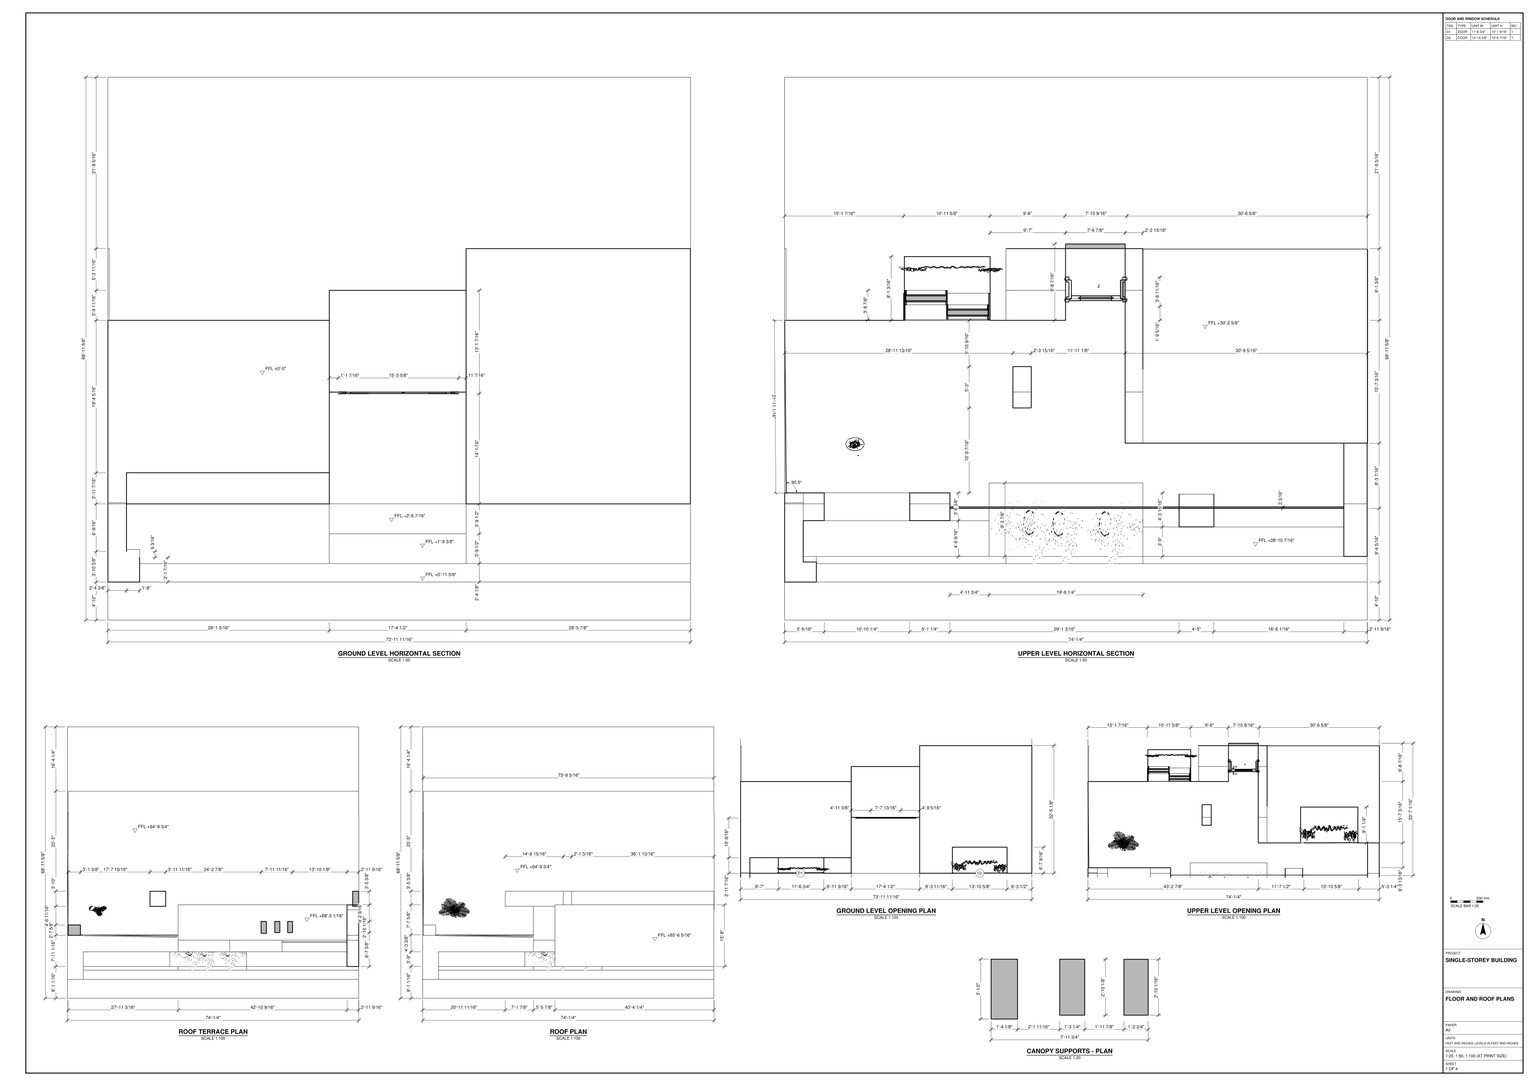
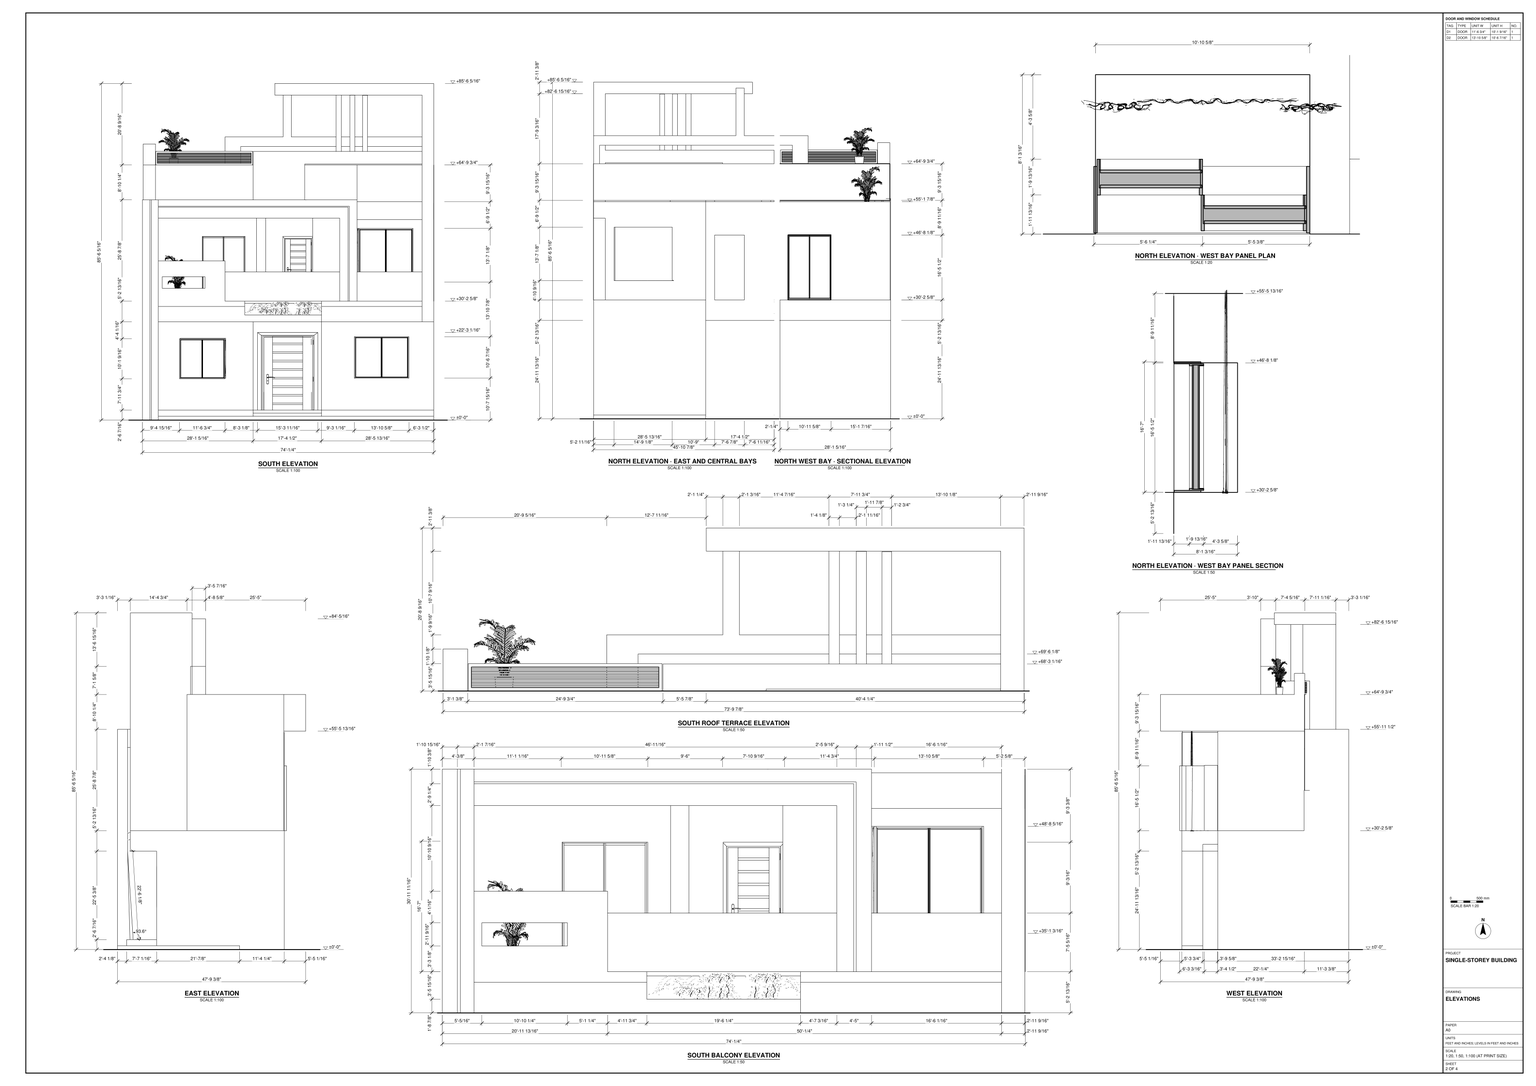
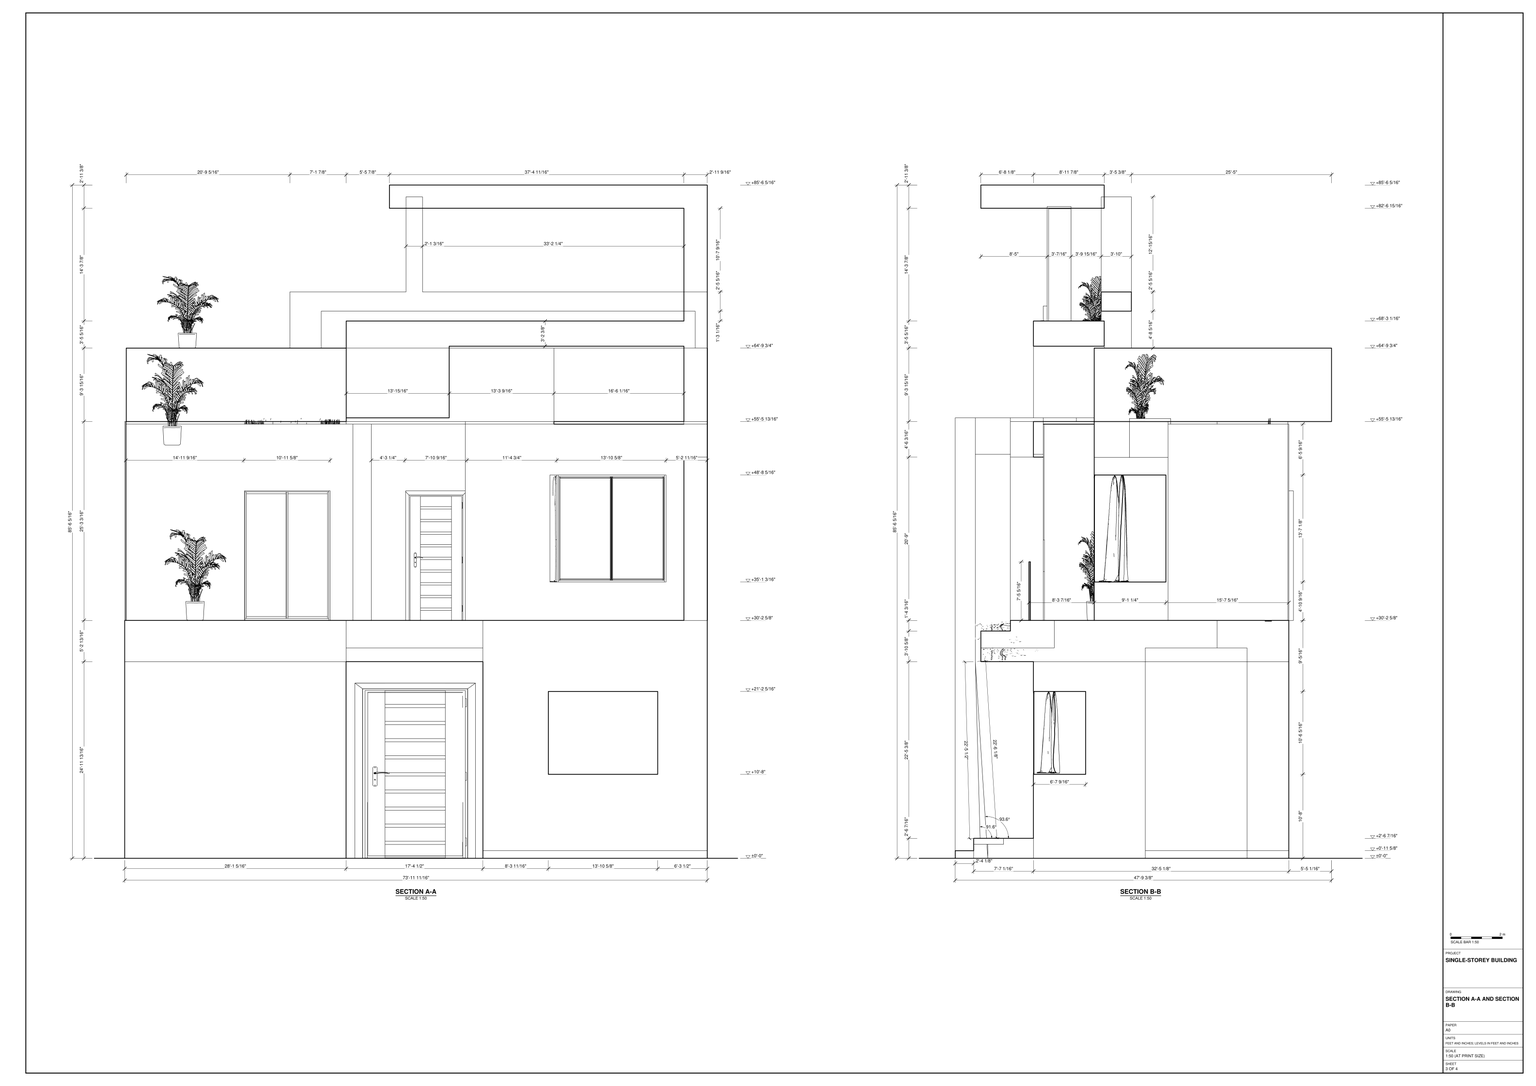
Build the house in SketchUp from task_files/diagram_01.pdf. Work in feet and inches, with the ground floor at ±0'-0". The overall model extents are 305'-8 9/16" along X, 356'-11 1/16" along Y and 85'-6 5/16" along Z. Use the dimensioned horizontal sections to lay out the building footprint and the setbacks between its bays.

Model the walls at the thicknesses drawn, the stepped entrance approach, the floor slabs and the flat roof. On the south elevation, place the framed entrance between the ground-floor windows. Above it, set the upper door and glazed openings behind the balcony. Follow the balcony detail for the projecting rectangular surround, the change in parapet height, the opening through the parapet and the planter above the entrance. Use the roof plan and sections to position the terrace parapet, horizontal screen and raised canopy with its slender supports.

Keep shell elements such as walls, slabs and roof, and each furniture or joinery piece, in separate groups or components; use components for repeated parts. Decor and loose items, including the terrace plants, may be any suitable library components, for example from 3D Warehouse. Save one SketchUp model as output_files/house_with_its_south_balcony_and_roof_terrace.skp.

# SketchUp Ruby script. Lengths in inches.
U = 1.inch
M = Sketchup.active_model
def pt(a) = Geom::Point3d.new(a.map { |v| v * U })
def face(e, loops, mat)
  f = e.add_face(loops[0].map { |a| pt(a) })
  loops[1..].each { |l| e.add_face(l.map { |a| pt(a) }).erase! }
  f.material = f.back_material = mat if mat
  f
end
# faces: each face lists its corners as indices into pts; further lists are holes
def faces(e, pts, list, mat = nil) = list.each { |f| face(e, (f[0].is_a?(Array) ? f : [f]).map { |l| l.map { |i| pts[i] } }, mat) }
# xy, xz, yz: faces in a plane at the given z, y or x. An outline is a flat list of corners, or four numbers for a rectangle; further outlines are holes
def ring(l) = l.size == 4 ? [[l[0], l[1]], [l[2], l[1]], [l[2], l[3]], [l[0], l[3]]] : l.each_slice(2).to_a
def flat(e, list, mat, &to3) = list.each { |f| face(e, (f[0].is_a?(Array) ? f : [f]).map { |l| ring(l).map { |u, v| to3.(u, v) } }, mat) }
def xy(e, z, list, mat = nil) = flat(e, list, mat) { |x, y| [x, y, z] }
def xz(e, y, list, mat = nil) = flat(e, list, mat) { |x, z| [x, y, z] }
def yz(e, x, list, mat = nil) = flat(e, list, mat) { |y, z| [x, y, z] }
def lines(e, pts, list) = list.each { |a, b| e.add_line(pt(pts[a]), pt(pts[b])) }
# prism: a flat outline (further loops are holes) pulled along v
def prism(e, loops, v, mat = nil)
  f = face(e, loops, mat); d = Geom::Vector3d.new(v.map { |x| x * U })
  f.pushpull(f.normal.samedirection?(d) ? d.length : -d.length)
end
def box(e, o, s, mat = nil) = prism(e, [[o, [o[0] + s[0], o[1], o[2]], [o[0] + s[0], o[1] + s[1], o[2]], [o[0], o[1] + s[1], o[2]]]], [0, 0, s[2]], mat)
def at(x, y, z, deg = 0) = Geom::Transformation.translation(pt([x, y, z])) * Geom::Transformation.rotation(ORIGIN, Z_AXIS, deg.degrees)
def axes(o, x, y, z) = Geom::Transformation.new([*x, 0, *y, 0, *z, 0, *pt(o).to_a, 1])
def part(name) = M.definitions.add(name)
# library, detail: a bought-in or finely detailed component or shape, given as its bounding box
def library(name, o, s) = part(name).tap { |d| box(d.entities, o, s) }
def detail(e, o, s) = box(e.add_group.entities, o, s)
def put(e, d, t, mat = nil) = e.add_instance(d, t).tap { |i| i.material = mat if mat }
def group(e, t, mat = nil) = e.add_group.tap { |g| g.transformation = t; g.material = mat if mat }.entities
root = M.entities
M.materials.add("Glass_Tinted_Gray").color = [0, 0, 0]
M.materials["Glass_Tinted_Gray"].alpha = 0.125
M.materials.add("Material~14").color = [247, 247, 247]
M.materials.add("Material~2").color = [49, 49, 49]
M.materials.add("Material~6").color = [130, 95, 63]
M.materials.add("Niraj_Hair_Dark").color = [109, 109, 109]
M.materials.add("[0135_DarkGray]").color = [81, 81, 81]
M.materials.add("[Asphalt_New]").color = [58, 58, 58]
M.materials.add("[Color C01]").color = [255, 229, 204]
M.materials.add("[Color M00]").color = [255, 255, 255]
M.materials.add("[Mirror 02]").color = [229, 229, 229]
M.materials.add("[Mirror 02]1").color = [229, 229, 229]
M.materials.add("[Terrazzo Light Blue]").color = [196, 214, 227]
c1 = library("curtian",[-4.5,-7.8,0.05],[158.46,10.43,112.21])
c2 = part("PENTEK_RP Fineline 50S_Sliding_DoorCase_E1")
box(c2.entities,[0,0,0],[1.51,3.66,99.27],"[0135_DarkGray]")
c3 = part("PENTEK_RP Fineline 50S_SlidingDooe_Case_E2")
box(c3.entities,[0,0,0],[96.25,3.66,1.51],"[0135_DarkGray]")
c4 = part("pentek_RP Fineline 50S_SlidingDoor_Case")
put(c4.entities,c2,at(97.76,0,0))
put(c4.entities,c3,at(1.51,0,0))
put(c4.entities,c2,at(0,0,0))
put(c4.entities,c3,at(1.51,0,97.76))
c5 = part("PENTEK_RP Fineline 50S_SlidingDoor_GlazingBead_2")
box(c5.entities,[0,0,0],[0.56,0.59,94.39],"[0135_DarkGray]")
c6 = part("PENTEK_RP Fineline 50S_SlidingDoor_Glass")
box(c6.entities,[0,0,0],[46.58,0.16,94.39],"Glass_Tinted_Gray")
c7 = part("PENTEK_RP Fineline 50S_SlidingDoor_GlazingBead")
box(c7.entities,[0,0,0],[45.47,0.59,0.56],"[0135_DarkGray]")
c8 = part("PENTEK_RP Fineline 50S_SlidingDoor_Leaf_E1")
xy(c8.entities,0,[[0,0,0.93,1.97],[0.93,1.57,1.49,1.97]],"[0135_DarkGray]")
xy(c8.entities,96.25,[[0,0,0.93,0,0.93,1.57,1.49,1.57,1.49,1.97,0,1.97]],"[0135_DarkGray]")
xz(c8.entities,0,[[0,0,0.93,96.25]],"[0135_DarkGray]")
xz(c8.entities,1.57,[[0.93,0,1.49,95.32],[0.93,95.32,1.49,96.25]],"[0135_DarkGray]")
xz(c8.entities,1.97,[[0,0,1.49,96.25]],"[0135_DarkGray]")
yz(c8.entities,0,[[0,0,1.97,96.25]],"[0135_DarkGray]")
yz(c8.entities,0.93,[[0,0,1.57,0.93],[0,0.93,1.57,95.32],[0,95.32,1.57,96.25]],"[0135_DarkGray]")
yz(c8.entities,1.49,[[1.57,0,1.97,95.32],[1.57,95.32,1.97,96.25]],"[0135_DarkGray]")
c9 = part("PENTEK_RP Fineline 50S_SlidingDoor_Leaf_E2")
xy(c9.entities,0,[[0,0,0,1.57,0.56,1.57,0.56,1.97,46.02,1.97,46.02,1.57,46.58,1.57,46.58,0]],"[0135_DarkGray]")
xy(c9.entities,0.93,[[0,0,46.58,1.57]],"[0135_DarkGray]")
xy(c9.entities,1.49,[[0.56,1.57,46.02,1.97]],"[0135_DarkGray]")
xz(c9.entities,0,[[0,0,46.58,0.93]],"[0135_DarkGray]")
xz(c9.entities,1.57,[[0,0,0.56,0.93],[46.02,0,46.58,0.93],[0.56,0.93,46.02,1.49]],"[0135_DarkGray]")
xz(c9.entities,1.97,[[0.56,0,46.02,1.49]],"[0135_DarkGray]")
yz(c9.entities,0,[[0,0,1.57,0.93]],"[0135_DarkGray]")
yz(c9.entities,0.56,[[1.57,0,1.97,0.93],[1.57,0.93,1.97,1.49]],"[0135_DarkGray]")
yz(c9.entities,46.02,[[1.57,0,1.97,0.93],[1.57,0.93,1.97,1.49]],"[0135_DarkGray]")
yz(c9.entities,46.58,[[0,0,1.57,0.93]],"[0135_DarkGray]")
c10 = part("PENTEK_RP Fineline S_SlidingDoor_Leaf1")
put(c10.entities,c5,at(0.93,0,0.93))
put(c10.entities,c5,at(46.96,0,0.93))
put(c10.entities,c6,at(1.49,1.42,0.93))
put(c10.entities,c7,at(1.49,0,0.93))
put(c10.entities,c6,at(1.49,0.59,0.93),"[Terrazzo Light Blue]")
put(c10.entities,c8,at(0,0,0))
put(c10.entities,c8,axes([48.44,0,0],[-1,0,0],[0,1,0],[0,0,1]))
put(c10.entities,c9,axes([0.93,0,96.25],[1,0,0],[0,1,0],[0,0,-1]))
put(c10.entities,c9,at(0.93,0,0))
put(c10.entities,c7,at(1.49,0,94.77))
c11 = part("PENTEK_RP Fineline 50S_SlidingDoor_Leaf2")
put(c11.entities,c6,at(1.49,1.42,0.93))
put(c11.entities,c7,at(1.49,0,94.77))
put(c11.entities,c5,at(46.96,0,0.93))
put(c11.entities,c6,at(1.49,0.59,0.93),"[Mirror 02]")
put(c11.entities,c5,at(0.93,0,0.93))
put(c11.entities,c8,at(0,0,0))
put(c11.entities,c8,axes([48.44,0,0],[-1,0,0],[0,1,0],[0,0,1]))
put(c11.entities,c7,at(1.49,0,0.93))
put(c11.entities,c9,axes([0.93,0,96.25],[1,0,0],[0,1,0],[0,0,-1]))
put(c11.entities,c9,at(0.93,0,0))
c12 = part("PENTEK - Slimmest Steel Sliding Door / Window\#1")
put(c12.entities,c4,at(0,-1.88,-0.09))
put(c12.entities,c10,at(1.51,-2.27,1.42))
put(c12.entities,c11,at(49.32,-0.3,1.42))
c13 = library("Group6\#1",[-22.44,-5.97,0],[42.52,9.29,84.25])
c14 = library("TS_VASO+GANCHOS-PARA-PENDURAR\#1",[-17.61,-15.74,-70.29],[36.55,50.24,77.96])
c15 = library("3D Plant 003",[-20.34,-12.34,-8.74],[41.02,24.08,18.2])
c16 = library("SKT_Nearly Natural 5' Kentia Palm Silk Tree",[-23.18,-17.61,0],[47.48,43.95,59.125])
c17 = part("Glass Door - Open Shower")
box(c17.entities,[0,0,0.95],[40,1.5,72])
c18 = part("Glass")
put(c18.entities,c17,axes([-0.67,0,24.24],[0,0,-0.606],[0,1,0],[0.69991,0,0]),"[Mirror 02]1")
c19 = library("Sphere Light",[-16.25,-16.25,-16.25],[32.5,32.5,32.5])
c20 = library("Sphere Light\#1",[-11.51,-11.51,-11.51],[23.02,23.02,23.02])
c21 = library("Sphere Light\#2",[-4.58,-4.58,-4.58],[9.16,9.16,9.16])
c22 = library("Sphere Light\#3",[-9.0625,-9.0625,-9.0625],[18.125,18.125,18.125])
c23 = library("Sphere Light\#4",[-6.43,-6.43,-6.43],[12.86,12.86,12.86])
c24 = library("Sphere Light\#5",[-6.71,-6.71,-6.71],[13.42,13.42,13.42])
c25 = library("Sphere Light\#6",[-9.57,-9.57,-9.57],[19.14,19.14,19.14])
c26 = library("Sphere Light\#7",[-21.77,-21.77,-21.77],[43.54,43.54,43.54])
c27 = library("Sphere Light\#8",[-25.16,-25.16,-25.16],[50.32,50.32,50.32])
c28 = library("Dome Light",[-12,-12,0],[24,24,12])
c29 = library("Dome Light\#1",[-12,-12,0],[24,24,12])
c30 = library("Dome Light\#2",[-12,-12,0],[24,24,12])
xy(root,0,[[0,0,3668.5625,4283.0625],[1460.375,2111.35,2348.05,2169.35],[1460.375,2169.35,2348.05,2169.35,2348.05,2677.67,2006.2,2677.67,2006.2,2288.52,1460.375,2288.52],[1460.375,2288.52,1488.72,2290.35],[1488.72,2288.52,1797.7,2288.52,1797.7,2568.29,1460.375,2568.29,1460.375,2290.35,1488.72,2290.35],
  [1797.7,2288.52,2006.2,2458.93],[1460.375,2568.29,1462.375,2677.67],[1462.375,2568.29,1797.7,2568.29,1797.7,2613.99,2006.2,2613.99,2006.2,2677.67,2348.05,2677.67,2348.05,2938.98,1460.375,2938.98,1460.375,2677.67,1462.375,2677.67]])
xy(root,11.625,[[1508.72,2169.35,2348.05,2197.47]])
xy(root,21.375,[[1797.7,2197.47,2006.2,2243]])
xy(root,30.4375,[[1508.72,2197.47,1797.7,2197.47,1797.7,2335.95,1488.72,2335.95,1488.72,2218.98,1508.72,2218.98],[2006.2,2197.47,2348.05,2288.52],[1797.7,2243,2006.2,2288.52]])
xy(root,128.03,[[1575.39,2288.52,1714.14,2335.95],[2105.92,2288.52,2272.54,2368.1]])
xy(root,249.53,[[1575.39,2288.52,1714.14,2335.95]])
xy(root,254.34,[[2105.92,2288.52,2272.54,2368.1]])
xy(root,299.8125,[[1488.72,2208.39,1797.7,2288.52],[1797.7,2208.39,2006.2,2677.67],[2006.2,2208.39,2068.96,2288.52],[2068.96,2208.39,2107.78,2288.52],[2107.78,2208.39,2348.05,2288.52],
  [1488.72,2288.52,1797.7,2335.95]])
xy(root,320.6875,[[1771.95,2208.39,2006.2,2320.29],[1797.7,2458.93,2006.2,2613.99]])
xy(root,346.43,[[1488.72,2208.39,1771.95,2262.95],[2006.2,2208.39,2312.46,2253.39]])
xy(root,362.625,[[[2006.2,2253.39,2061.4,2253.39,2061.4,2303.45,2114.41,2303.45,2114.41,2253.39,2312.46,2253.39,2312.46,2381.11,1979.26,2381.11,1979.26,2684.73,1888.39,2684.73,1888.39,2568.29,1460.375,2568.29,1462.74,2305.32,1712.19,2305.32,1712.19,2262.95,1771.95,2262.95,1771.95,2320.29,2006.2,2320.29],[1808.19,2434.75,1836.13,2497.75]],[2061.4,2253.39,2114.41,2303.45],[1460.375,2305.32,1462.74,2305.32,1460.375,2568.29],[2006.2,2381.11,2348.05,2676.24],[2348.05,2381.11,2348.61,2676.24],
  [1642.8,2568.29,1773.42,2665.48],[2006.2,2676.24,2348.05,2677.67]])
xy(root,401.75,[[1520.68,2262.95,1650.9375,2305.32]])
xy(root,421.2,[[2108.27,2381.11,2282.83,2490.36]])
xy(root,437.25,[[1520.68,2262.95,1650.9375,2305.32]])
xy(root,485.3125,[[1488.72,2262.95,1712.19,2262.95,1712.19,2305.32,1460.375,2305.32,1460.375,2290.35,1488.72,2290.35],[1460.375,2288.52,1488.72,2290.35]])
xy(root,560.12,[[1642.8,2568.29,1773.42,2665.48],[1888.39,2568.29,1979.26,2684.73]])
xy(root,584.33,[[2108.27,2381.11,2282.83,2490.36]])
xy(root,611.61,[[2114.41,2288.52,2312.46,2303.45]])
xy(root,661.875,[[2114.41,2303.45,2312.46,2381.11],[1979.26,2493.62,2006.2,2493.62,2006.2,2677.67,1797.7,2677.67,1797.7,2568.29,1979.26,2568.29]])
xy(root,665.8125,[[2114.41,2288.52,2312.46,2381.11],[1462.75,2304.74,1462.75,2742.74,2348.05,2742.74,2348.05,2381.11,1797.9,2381.11,1797.9,2304.74]])
xy(root,670.375,[[1808.19,2434.75,1836.13,2497.75]])
xy(root,671.5,[[1460.375,2169.35,1460.375,2303.45,1797.9,2303.45,1797.9,2253.39,1508.72,2253.39,1508.72,2169.35],[1797.9,2253.39,1954.84,2288.52],[1954.84,2253.39,2114.41,2303.45],[1797.9,2288.52,1954.84,2303.45],[1797.9,2303.45,1954.84,2381.11]])
xy(root,777.75,[[1796.3,2299.59,1501.21,2304.74,1509.71,2304.74,1796.3,2299.73],[1462.75,2303.45,1500.15,2303.45,1462.75,2304.74],[1500.15,2303.45,1462.75,2304.74,1500.15,2304.74],[[1500.15,2304.74,1501.21,2304.74,1501.22,2304.89,1509.71,2304.74,1797.9,2304.74,1797.9,2396.36,1954.84,2396.36,1954.84,2381.11,2312.46,2381.11,2312.46,2396.36,2348.05,2396.36,2348.05,2384.86,2348.61,2384.86,2348.61,2676.24,2348.05,2676.24,2348.05,2742.74,1462.75,2742.74,1462.75,2335.05,1500.15,2335.05],[1712.05,2391.77,1759.8,2437.77]],[1501.21,2304.74,1501.22,2304.89,1509.71,2304.74],
  [1797.9,2381.11,1954.84,2396.36],[2312.46,2381.11,2348.05,2396.36],[2348.05,2381.11,2348.61,2384.86]])
xy(root,777.77,[[2329.69,2391.77,2348.05,2437.77]])
xy(root,780.6875,[[1954.84,2288.52,2312.46,2396.36]])
xy(root,782.77,[[1791.87,2299.66,1791.875,2299.96,1505.64,2304.96,1505.64,2304.66]])
xy(root,782.77,[[1791.83,2297.14,1791.87,2299.66,1505.64,2304.66,1505.6,2302.14]],"Material~2")
xy(root,783.44,[[1791.23,2297.15,1506.19,2302.13,1506.23,2304.8,1791.28,2299.82]],"Material~2")
xy(root,785.24,[[1791.25,2298,1791.28,2299.82,1506.23,2304.8,1506.2,2302.98]],"Material~2")
xy(root,787.03,[[1791.25,2298,1506.2,2302.98,1506.23,2304.8,1791.28,2299.82]],"Material~2")
xy(root,788.82,[[1791.25,2298,1791.28,2299.82,1506.23,2304.8,1506.2,2302.98]],"Material~2")
xy(root,790.62,[[1791.25,2298,1506.2,2302.98,1506.23,2304.8,1791.28,2299.82]],"Material~2")
xy(root,792.41,[[1791.25,2298,1791.28,2299.82,1506.23,2304.8,1506.2,2302.98]],"Material~2")
xy(root,794.2,[[1791.25,2298,1506.2,2302.98,1506.23,2304.8,1791.28,2299.82]],"Material~2")
xy(root,796,[[1791.25,2298,1791.28,2299.82,1506.23,2304.8,1506.2,2302.98]],"Material~2")
xy(root,797.79,[[1791.25,2298,1506.2,2302.98,1506.23,2304.8,1791.28,2299.82]],"Material~2")
xy(root,799.58,[[1791.25,2298,1791.28,2299.82,1506.23,2304.8,1506.2,2302.98]],"Material~2")
xy(root,801.375,[[1791.25,2298,1506.2,2302.98,1506.23,2304.8,1791.28,2299.82]],"Material~2")
xy(root,803.17,[[1791.25,2298,1791.28,2299.82,1506.23,2304.8,1506.2,2302.98]],"Material~2")
xy(root,804.96,[[1791.25,2298,1506.2,2302.98,1506.23,2304.8,1791.28,2299.82]],"Material~2")
xy(root,806.76,[[1791.25,2298,1791.28,2299.82,1506.23,2304.8,1506.2,2302.98]],"Material~2")
xy(root,808.55,[[1791.25,2298,1506.2,2302.98,1506.23,2304.8,1791.28,2299.82]],"Material~2")
xy(root,810.34,[[1791.25,2298,1791.28,2299.82,1506.23,2304.8,1506.2,2302.98]],"Material~2")
xy(root,812.13,[[1791.25,2298,1506.2,2302.98,1506.23,2304.8,1791.28,2299.82]],"Material~2")
xy(root,813.93,[[1791.23,2297.15,1791.28,2299.82,1506.23,2304.8,1506.19,2302.13]],"Material~2")
xy(root,814.6,[[1791.87,2299.66,1505.64,2304.66,1505.64,2304.96,1791.875,2299.96]])
xy(root,814.6,[[1791.83,2297.14,1505.6,2302.14,1505.64,2304.66,1791.87,2299.66]],"Material~2")
xy(root,819.05,[[[1797.9,2288.52,2312.46,2396.36],[2050.64,2309.39,2066.76,2345.89],[2092.45,2311.77,2107.7,2345.89],[2131.62,2311.77,2146.37,2345.83]]])
xy(root,819.62,[[1796.3,2299.59,1796.3,2299.73,1501.22,2304.89,1501.21,2304.74]])
xy(root,834.09,[[1759.8,2391.77,2329.69,2437.77]])
xy(root,841.875,[[1462.75,2303.45,1500.15,2335.05]])
xy(root,863.375,[[1712.05,2391.77,1889.02,2437.77],[1914.2,2391.77,2348.05,2437.77]])
xy(root,990.23,[[2131.62,2311.77,2146.37,2345.83]])
xy(root,990.61,[[2092.45,2311.77,2107.7,2345.89]])
xy(root,990.94,[[1863.78,2208.39,2312.46,2396.36]])
xy(root,993.73,[[2050.64,2309.39,2066.76,2345.89]])
xy(root,1008.3125,[[1889.02,2391.77,1914.2,2437.77]])
xy(root,1026.3125,[[1863.78,2208.39,2348.05,2396.36]])
xz(root,2169.35,[[1483.3,0,1487.83,671.5]])
xz(root,2169.35,[[1460.375,0,1483.3,671.5],[1487.83,0,1508.72,671.5]],"Material~6")
xz(root,2169.35,[[1508.72,0,2348.05,11.625]],"[Color M00]")
xz(root,2197.47,[[1797.7,0,2006.2,11.625],[1508.72,11.625,1797.7,30.4375],[1797.7,11.625,2006.2,21.375],[2006.2,11.625,2348.05,30.4375]])
xz(root,2199.93,[[1488.72,299.8125,1508.72,615.9]])
xz(root,2208.39,[[2312.46,299.8125,2348.05,299.8125,2348.05,1026.3125,1863.78,1026.3125,1863.78,990.94,2312.46,990.94]])
xz(root,2208.39,[[1488.72,299.8125,2006.2,299.8125,2006.2,320.6875,1771.95,320.6875,1771.95,346.43,1488.72,346.43],[2006.2,299.8125,2312.46,346.43]],"Niraj_Hair_Dark")
xz(root,2218.98,[[1488.72,0,1508.72,30.4375]])
xz(root,2243,[[1797.7,21.375,2006.2,30.4375]])
xz(root,2253.39,[[2006.2,346.43,2312.46,362.625],[2087.16,362.625,2090.9375,362.625,2090.9375,651.9375,1508.72,651.9375,1508.72,649.15,2087.16,649.15]])
xz(root,2253.39,[[2061.4,362.625,2087.16,362.625,2087.16,649.15,1508.72,649.15,1508.72,615.9,2061.4,615.9],[2090.9375,362.625,2114.41,362.625,2114.41,671.5,1508.72,671.5,1508.72,651.9375,2090.9375,651.9375]],"Material~6")
xz(root,2262.95,[[[1488.72,346.43,1771.95,346.43,1771.95,362.625,1712.19,362.625,1712.19,485.3125,1488.72,485.3125],[1520.68,401.75,1650.9375,437.25]]])
xz(root,2288.52,[[1797.7,0,1814.75,11.625],[1814.75,0,2006.2,11.625],[[1488.72,11.625,1797.7,299.8125],[1575.39,128.03,1714.14,249.53]],[1797.7,11.625,2006.2,30.4375],[2114.41,611.61,2312.46,665.8125],
  [1797.9,671.5,1954.84,671.5,1954.84,780.6875,2312.46,780.6875,2312.46,819.05,1797.9,819.05]])
xz(root,2288.52,[[[2006.2,30.4375,2348.05,299.8125],[2105.92,128.03,2272.54,254.34]]],"[Color C01]")
xz(root,2303.45,[[1460.375,615.9,1462.375,671.5],[2114.41,665.8125,2114.41,671.5,1954.84,671.5],[1462.75,777.75,1500.15,841.875]])
xz(root,2304.74,[[1462.75,665.8125,1797.9,777.75]],"Niraj_Hair_Dark")
xz(root,2305.32,[[[1460.375,362.625,1712.19,485.3125],[1520.68,401.75,1650.9375,437.25]]])
xz(root,2309.39,[[2050.64,819.05,2066.76,993.73]])
xz(root,2311.77,[[2092.45,819.05,2107.7,990.61],[2131.62,819.05,2146.37,990.23]])
xz(root,2320.29,[[1771.95,320.6875,2006.2,356.29],[1771.95,356.29,2006.2,362.625]])
xz(root,2335.05,[[1462.75,777.75,1500.15,841.875]])
xz(root,2335.95,[[[1488.72,30.4375,1797.7,299.8125],[1575.39,128.03,1714.14,249.53]],[1575.39,128.03,1714.14,249.53]])
xz(root,2345.83,[[2131.62,819.05,2146.37,990.23]])
xz(root,2345.89,[[2050.64,819.05,2066.76,993.73],[2092.45,819.05,2107.7,990.61]])
xz(root,2368.1,[[2105.92,128.03,2272.54,254.34]])
xz(root,2381.11,[[[1979.26,362.625,2312.46,362.625,2312.46,611.61,2347.97,611.61,2347.97,661.875,1979.26,661.875],[2108.27,421.2,2282.83,584.33]],[2312.46,362.625,2348.05,611.61],[2348.05,362.625,2348.61,611.61],[2347.97,611.61,2348.05,661.875],[2348.05,611.61,2348.61,661.875],
  [1797.9,661.875,1979.26,665.8125],[1979.26,661.875,2114.41,665.8125],[2114.41,661.875,2312.46,665.8125],[2312.46,661.875,2348.05,777.75],[2348.05,661.875,2348.61,665.8125],
  [2348.05,665.8125,2348.61,777.75],[1797.9,671.5,1954.84,777.75]])
xz(root,2381.11,[[2114.41,665.8125,2312.46,777.75]],"Material~6")
xz(root,2381.11,[[1797.9,665.8125,2114.41,665.8125,2114.41,777.75,1954.84,777.75,1954.84,671.5,1797.9,671.5]],"Niraj_Hair_Dark")
xz(root,2391.77,[[1712.05,777.75,1759.8,777.75,1759.8,834.09,2329.69,834.09,2329.69,777.77,2348.05,777.77,2348.05,863.375,1914.2,863.375,1914.2,1008.3125,1889.02,1008.3125,1889.02,863.375,1712.05,863.375]],"Niraj_Hair_Dark")
xz(root,2396.36,[[1797.9,777.75,1797.9,819.05,2312.46,819.05,2312.46,990.94,1863.78,990.94,1863.78,1026.3125,2348.05,1026.3125,2348.05,777.75,2312.46,777.75,2312.46,780.6875,1954.84,780.6875,1954.84,777.75]])
xz(root,2434.75,[[1808.19,362.625,1836.13,670.375]])
xz(root,2437.77,[[1712.05,777.75,1712.05,863.375,1889.02,863.375,1889.02,1008.3125,1914.2,1008.3125,1914.2,863.375,2348.05,863.375,2348.05,777.77,2329.69,777.77,2329.69,834.09,1759.8,834.09,1759.8,777.75]])
xz(root,2458.93,[[1797.7,0,2006.2,320.6875]])
xz(root,2490.36,[[2108.27,421.2,2282.83,584.33]])
xz(root,2493.62,[[1979.26,611.0625,2006.2,661.875]])
xz(root,2497.75,[[1808.19,362.625,1836.13,670.375]])
xz(root,2568.29,[[1460.375,0,1797.7,299.8125],[1460.375,299.8125,1797.7,362.625]])
xz(root,2568.29,[[1462.375,362.625,1642.8,362.625,1642.8,560.12,1773.42,560.12,1773.42,362.625,1888.39,362.625,1888.39,560.12,1979.26,560.12,1979.26,661.875,1462.375,661.875]],"[Color C01]")
xz(root,2613.99,[[1797.7,0,2006.2,320.6875]])
xz(root,2665.48,[[1642.8,362.625,1773.42,560.12]])
xz(root,2676.24,[[2348.05,362.625,2348.61,665.8125],[2348.05,665.8125,2348.61,777.75]])
xz(root,2677.67,[[2006.2,0,2348.05,11.625],[2006.2,11.625,2348.05,362.625],[1797.7,299.8125,2006.2,661.875]])
xz(root,2684.73,[[1888.39,362.625,1979.26,560.12]])
xz(root,2742.74,[[1462.75,665.8125,2348.05,777.75]])
yz(root,1460.375,[[2169.35,0,2169.35,671.5,2303.45,671.5,2303.45,485.3125,2305.32,485.3125,2305.32,362.625,2568.29,362.625,2568.29,0]],"Material~14")
yz(root,1462.75,[[2304.74,665.8125,2304.74,777.75,2303.45,777.75,2303.45,841.875,2335.05,841.875,2335.05,777.75,2742.74,777.75,2742.74,665.8125]])
yz(root,1488.72,[[2288.52,0,2290.35,11.625],[2288.52,11.625,2290.35,30.4375],[2288.52,30.4375,2335.95,299.8125]])
yz(root,1488.72,[[2218.98,0,2218.98,30.4375,2288.52,30.4375,2288.52,299.8125,2208.39,299.8125,2208.39,346.43,2262.95,346.43,2262.95,485.3125,2288.52,485.3125,2288.52,615.9,2199.93,615.9,2199.93,299.8125]],"Niraj_Hair_Dark")
yz(root,1500.15,[[2303.45,777.75,2335.05,841.875]])
yz(root,1505.64,[[2304.66,782.77,2304.96,814.6]])
yz(root,1506.2,[[2302.83,785.24,2302.83,785.57,2302.875,785.34,2302.98,785.24],[2302.83,786.7,2302.83,787.03,2302.98,787.03,2302.875,786.93],[2302.83,788.82,2302.83,789.16,2302.875,788.92,2302.98,788.82],[2302.83,790.28,2302.83,790.62,2302.98,790.62,2302.875,790.52],[2302.83,792.41,2302.83,792.75,2302.875,792.51,2302.98,792.41],
  [2302.83,793.87,2302.83,794.2,2302.98,794.2,2302.875,794.11],[2302.83,796,2302.83,796.33,2302.875,796.09,2302.98,796],[2302.83,797.45,2302.83,797.79,2302.98,797.79,2302.875,797.69],[2302.83,799.58,2302.83,799.92,2302.875,799.68,2302.98,799.58],[2302.83,801.04,2302.83,801.375,2302.98,801.375,2302.875,801.28],
  [2302.83,803.17,2302.83,803.5,2302.875,803.27,2302.98,803.17],[2302.83,804.625,2302.83,804.96,2302.98,804.96,2302.875,804.86],[2302.83,806.76,2302.83,807.09,2302.875,806.85,2302.98,806.76],[2302.83,808.21,2302.83,808.55,2302.98,808.55,2302.875,808.45],[2302.83,810.34,2302.83,810.68,2302.875,810.4375,2302.98,810.34],
  [2302.83,811.8,2302.83,812.13,2302.98,812.13,2302.875,812.04]])
yz(root,1508.72,[[2197.47,0,2218.98,0,2217.04,30.4375,2197.47,30.4375],[2218.98,0,2217.04,30.4375,2218.98,30.4375]])
yz(root,1508.72,[[2169.35,11.625,2197.47,11.625,2197.47,30.4375,2207.26,30.4375,2199.93,299.8125,2199.93,671.5,2169.35,671.5],[2199.93,615.9,2253.39,671.5]],"Material~6")
yz(root,1520.68,[[2262.95,401.75,2305.32,437.25]])
yz(root,1575.39,[[2288.52,128.03,2335.95,249.53]])
yz(root,1642.8,[[2568.29,362.625,2665.48,560.12]])
yz(root,1650.9375,[[2262.95,401.75,2305.32,437.25]])
yz(root,1712.05,[[2391.77,777.75,2437.77,863.375]])
yz(root,1712.19,[[2262.95,362.625,2305.32,437.25],[2262.95,437.25,2305.32,485.3125]])
yz(root,1714.14,[[2288.52,128.03,2335.95,249.53]])
yz(root,1759.8,[[2391.77,777.75,2437.77,834.09]])
yz(root,1771.95,[[2208.39,320.6875,2320.29,320.6875,2320.29,356.29,2262.95,356.29,2262.95,346.43,2208.39,346.43],[2262.95,356.29,2320.29,362.625]])
yz(root,1773.42,[[2568.29,362.625,2665.48,560.12]])
yz(root,1791.25,[[2297.86,785.24,2298,785.24,2297.9,785.34,2297.86,785.57],[2297.86,786.7,2297.9,786.93,2298,787.03,2297.86,787.03],[2297.86,788.82,2298,788.82,2297.9,788.92,2297.86,789.16],[2297.86,790.28,2297.9,790.52,2298,790.62,2297.86,790.62],[2297.86,792.41,2298,792.41,2297.9,792.51,2297.86,792.75],
  [2297.86,793.87,2297.9,794.11,2298,794.2,2297.86,794.2],[2297.86,796,2298,796,2297.9,796.09,2297.86,796.33],[2297.86,797.45,2297.9,797.69,2298,797.79,2297.86,797.79],[2297.86,799.58,2298,799.58,2297.9,799.68,2297.86,799.92],[2297.86,801.04,2297.9,801.28,2298,801.375,2297.86,801.375],
  [2297.86,803.17,2298,803.17,2297.9,803.27,2297.86,803.5],[2297.86,804.625,2297.9,804.86,2298,804.96,2297.86,804.96],[2297.86,806.76,2298,806.76,2297.9,806.85,2297.86,807.09],[2297.86,808.21,2297.9,808.45,2298,808.55,2297.86,808.55],[2297.86,810.34,2298,810.34,2297.9,810.4375,2297.86,810.68],
  [2297.86,811.8,2297.9,812.04,2298,812.13,2297.86,812.13]])
yz(root,1796.3,[[2299.59,777.75,2299.73,819.62]])
yz(root,1797.7,[[2288.52,0,2458.93,0,2458.93,299.8125,2335.95,299.8125,2335.95,30.4375,2288.52,30.4375],[2458.93,0,2568.29,299.8125],[2568.29,0,2613.99,299.8125],[2197.47,21.375,2243,30.4375],[2288.52,30.4375,2335.95,290],
  [2288.52,290,2335.95,299.8125],[2458.93,299.8125,2568.29,320.6875],[2568.29,299.8125,2613.99,320.6875]])
yz(root,1797.9,[[2304.74,665.8125,2381.11,671.5],[2288.52,671.5,2288.52,819.05,2396.36,819.05,2396.36,777.75,2304.74,777.75,2304.74,671.5],[2304.74,671.5,2381.11,777.75]])
yz(root,1808.19,[[2434.75,362.625,2497.75,670.375]])
yz(root,1836.13,[[2434.75,362.625,2497.75,670.375]])
yz(root,1863.78,[[2208.39,990.94,2396.36,1026.3125]])
yz(root,1888.39,[[2568.29,362.625,2684.73,560.12]])
yz(root,1889.02,[[2391.77,863.375,2437.77,1008.3125]])
yz(root,1914.2,[[2391.77,863.375,2437.77,1008.3125]])
yz(root,1954.84,[[2288.52,671.5,2381.11,671.5,2381.11,777.75,2396.36,777.75,2396.36,780.6875,2288.52,780.6875]])
yz(root,1979.26,[[2381.11,362.625,2381.11,611.0625,2493.62,611.0625,2493.62,661.875,2568.29,661.875,2568.29,560.12,2684.73,560.12,2684.73,362.625]])
yz(root,2006.2,[[2288.52,0,2458.93,299.8125],[2458.93,0,2613.99,11.625],[2613.99,0,2677.67,11.625],[2458.93,11.625,2613.99,299.8125],[2613.99,11.625,2677.67,299.8125],
  [2197.47,21.375,2243,30.4375],[2458.93,299.8125,2613.99,320.6875],[2208.39,320.6875,2208.39,346.43,2253.39,346.43,2253.39,362.625,2320.29,362.625,2320.29,320.6875],[2493.62,362.625,2676.24,661.875],[2676.24,362.625,2677.67,661.875]])
yz(root,2050.64,[[2309.39,819.05,2345.89,993.73]])
yz(root,2061.4,[[2253.39,362.625,2303.45,615.9]],"Material~6")
yz(root,2066.76,[[2309.39,819.05,2345.89,993.73]])
yz(root,2092.45,[[2311.77,819.05,2345.89,990.61]])
yz(root,2105.92,[[2288.52,128.03,2368.1,254.34]])
yz(root,2107.7,[[2311.77,819.05,2345.89,990.61]])
yz(root,2108.27,[[2381.11,421.2,2490.36,584.33]])
yz(root,2114.41,[[2253.39,362.625,2303.45,611.61],[2253.39,611.61,2288.52,665.8125],[2303.45,661.875,2381.11,665.8125],[2253.39,665.8125,2303.45,671.5]])
yz(root,2131.62,[[2311.77,819.05,2345.83,990.23]])
yz(root,2146.37,[[2311.77,819.05,2345.83,990.23]])
yz(root,2272.54,[[2288.52,128.03,2368.1,254.34]])
yz(root,2282.83,[[2381.11,421.2,2490.36,584.33]])
yz(root,2312.46,[[2208.39,346.43,2208.39,990.94,2396.36,990.94,2396.36,819.05,2288.52,819.05,2288.52,780.6875,2396.36,780.6875,2396.36,777.75,2381.11,777.75,2381.11,665.8125,2288.52,665.8125,2288.52,611.61,2381.11,611.61,2381.11,362.625,2253.39,362.625,2253.39,346.43]])
yz(root,2329.69,[[2391.77,777.77,2437.77,834.09]])
yz(root,2348.05,[[2169.35,0,2541.42,11.625],[2541.42,0,2677.67,0,2677.67,362.625,2208.39,362.625,2208.39,299.8125,2288.52,299.8125,2288.52,11.625,2541.42,11.625],[2197.47,11.625,2288.52,30.4375],[2208.39,362.625,2381.11,362.625,2381.11,777.75,2396.36,777.75,2396.36,777.77,2391.77,777.77,2391.77,863.375,2396.36,863.375,2396.36,1026.3125,2208.39,1026.3125],[2676.24,665.8125,2742.74,777.75],
  [2391.77,777.77,2396.36,863.375],[2396.36,777.77,2437.77,863.375]])
yz(root,2348.61,[[2381.11,362.625,2676.24,777.75]])
p = [[1462.74,2305.32,362.625],[1460.375,2568.29,362.625],[1460.375,2568.29,665.8125],[1462.75,2304.74,665.8125],[1462.75,2304.74,362.625],[2114.41,2303.45,665.8125],
  [1954.84,2303.45,671.5],[1954.84,2353.95,671.5],[2114.41,2353.95,665.8125],[1500.15,2303.45,777.75],[1462.75,2304.74,777.75],[1462.75,2304.74,671.5],
  [1500.15,2303.45,671.5],[1796.3,2299.59,819.62],[1501.21,2304.74,819.62],[1501.21,2304.74,777.75],[1796.3,2299.59,777.75],[1791.87,2299.66,782.77],
  [1505.64,2304.66,782.77],[1505.64,2304.66,814.6],[1791.87,2299.66,814.6],[1501.3,2304.99,777.85],[1796.21,2299.84,777.85],[1796.3,2299.73,777.75],
  [1509.71,2304.74,777.75],[1501.22,2304.89,777.75],[1796.21,2299.84,819.52],[1796.3,2299.73,819.62],[1501.51,2305.03,778.08],[1796.01,2299.89,778.08],
  [1796.01,2299.89,819.29],[1501.22,2304.89,819.62],[1501.3,2304.99,819.52],[1501.51,2305.03,819.29],[1791.875,2299.96,782.77],[1791.875,2299.96,814.6],
  [1505.64,2304.96,814.6],[1505.64,2304.96,782.77],[1505.68,2302.03,782.87],[1791.74,2297.04,782.87],[1791.83,2297.14,782.77],[1505.6,2302.14,782.77],
  [1791.74,2297.04,814.5],[1791.83,2297.14,814.6],[1505.9375,2304.95,811.8],[1791.58,2299.97,811.8],[1791.58,2299.97,814.26],[1505.9375,2304.95,814.26],
  [1791.58,2299.97,801.04],[1791.58,2299.97,803.5],[1505.9375,2304.95,803.5],[1505.9375,2304.95,801.04],[1791.58,2299.97,783.11],[1791.58,2299.97,785.57],
  [1505.9375,2304.95,785.57],[1505.9375,2304.95,783.11],[1791.58,2299.97,786.7],[1791.58,2299.97,789.16],[1505.9375,2304.95,789.16],[1505.9375,2304.95,786.7],
  [1791.58,2299.97,793.87],[1791.58,2299.97,796.33],[1505.9375,2304.95,796.33],[1505.9375,2304.95,793.87],[1505.9375,2304.95,799.92],[1505.9375,2304.95,797.45],
  [1791.58,2299.97,797.45],[1791.58,2299.97,799.92],[1791.58,2299.97,808.21],[1791.58,2299.97,810.68],[1505.9375,2304.95,810.68],[1505.9375,2304.95,808.21],
  [1505.9375,2304.95,804.625],[1791.58,2299.97,804.625],[1791.58,2299.97,807.09],[1505.9375,2304.95,807.09],[1791.58,2299.97,792.75],[1505.9375,2304.95,792.75],
  [1505.9375,2304.95,790.28],[1791.58,2299.97,790.28],[1505.68,2302.03,814.5],[1505.6,2302.14,814.6],[1505.89,2301.99,783.11],[1791.53,2297,783.11],
  [1791.53,2297,814.26],[1505.89,2301.99,814.26],[1506.1,2302.03,783.35],[1791.32,2297.05,783.35],[1791.32,2297.05,814.03],[1506.15,2304.9,783.35],
  [1791.37,2299.93,783.35],[1791.37,2299.93,785.34],[1506.1,2302.03,814.03],[1506.15,2304.9,785.34],[1506.19,2302.13,783.44],[1791.23,2297.15,783.44],
  [1791.23,2297.15,813.93],[1791.28,2299.82,783.44],[1506.23,2304.8,783.44],[1791.28,2299.82,785.24],[1506.19,2302.13,813.93],[1506.23,2304.8,785.24],
  [1791.28,2299.82,813.93],[1791.25,2298,785.24],[1791.25,2297.86,785.24],[1791.25,2297.86,785.57],[1791.25,2297.86,786.7],[1791.25,2297.86,787.03],
  [1791.25,2298,787.03],[1791.28,2299.82,787.03],[1791.28,2299.82,788.82],[1791.25,2298,788.82],[1791.25,2297.86,788.82],[1791.25,2297.86,789.16],
  [1791.25,2297.86,790.28],[1791.25,2297.86,790.62],[1791.25,2298,790.62],[1791.28,2299.82,790.62],[1791.28,2299.82,792.41],[1791.25,2298,792.41],
  [1791.25,2297.86,792.41],[1791.25,2297.86,792.75],[1791.25,2297.86,793.87],[1791.25,2297.86,794.2],[1791.25,2298,794.2],[1791.28,2299.82,794.2],
  [1791.28,2299.82,796],[1791.25,2298,796],[1791.25,2297.86,796],[1791.25,2297.86,796.33],[1791.25,2297.86,797.45],[1791.25,2297.86,797.79],
  [1791.25,2298,797.79],[1791.28,2299.82,797.79],[1791.28,2299.82,799.58],[1791.25,2298,799.58],[1791.25,2297.86,799.58],[1791.25,2297.86,799.92],
  [1791.25,2297.86,801.04],[1791.25,2297.86,801.375],[1791.25,2298,801.375],[1791.28,2299.82,801.375],[1791.28,2299.82,803.17],[1791.25,2298,803.17],
  [1791.25,2297.86,803.17],[1791.25,2297.86,803.5],[1791.25,2297.86,804.625],[1791.25,2297.86,804.96],[1791.25,2298,804.96],[1791.28,2299.82,804.96],
  [1791.28,2299.82,806.76],[1791.25,2298,806.76],[1791.25,2297.86,806.76],[1791.25,2297.86,807.09],[1791.25,2297.86,808.21],[1791.25,2297.86,808.55],
  [1791.25,2298,808.55],[1791.28,2299.82,808.55],[1791.28,2299.82,810.34],[1791.25,2298,810.34],[1791.25,2297.86,810.34],[1791.25,2297.86,810.68],
  [1791.25,2297.86,811.8],[1791.25,2297.86,812.13],[1791.25,2298,812.13],[1791.28,2299.82,812.13],[1506.23,2304.8,813.93],[1506.23,2304.8,812.13],
  [1506.2,2302.98,812.13],[1506.2,2302.83,812.13],[1506.2,2302.83,811.8],[1506.2,2302.83,810.68],[1506.2,2302.83,810.34],[1506.2,2302.98,810.34],
  [1506.23,2304.8,810.34],[1506.23,2304.8,808.55],[1506.2,2302.98,808.55],[1506.2,2302.83,808.55],[1506.2,2302.83,808.21],[1506.2,2302.83,807.09],
  [1506.2,2302.83,806.76],[1506.2,2302.98,806.76],[1506.23,2304.8,806.76],[1506.23,2304.8,804.96],[1506.2,2302.98,804.96],[1506.2,2302.83,804.96],
  [1506.2,2302.83,804.625],[1506.2,2302.83,803.5],[1506.2,2302.83,803.17],[1506.2,2302.98,803.17],[1506.23,2304.8,803.17],[1506.23,2304.8,801.375],
  [1506.2,2302.98,801.375],[1506.2,2302.83,801.375],[1506.2,2302.83,801.04],[1506.2,2302.83,799.92],[1506.2,2302.83,799.58],[1506.2,2302.98,799.58],
  [1506.23,2304.8,799.58],[1506.23,2304.8,797.79],[1506.2,2302.98,797.79],[1506.2,2302.83,797.79],[1506.2,2302.83,797.45],[1506.2,2302.83,796.33],
  [1506.2,2302.83,796],[1506.2,2302.98,796],[1506.23,2304.8,796],[1506.23,2304.8,794.2],[1506.2,2302.98,794.2],[1506.2,2302.83,794.2],
  [1506.2,2302.83,793.87],[1506.2,2302.83,792.75],[1506.2,2302.83,792.41],[1506.2,2302.98,792.41],[1506.23,2304.8,792.41],[1506.23,2304.8,790.62],
  [1506.2,2302.98,790.62],[1506.2,2302.83,790.62],[1506.2,2302.83,790.28],[1506.2,2302.83,789.16],[1506.2,2302.83,788.82],[1506.2,2302.98,788.82],
  [1506.23,2304.8,788.82],[1506.23,2304.8,787.03],[1506.2,2302.98,787.03],[1506.2,2302.83,787.03],[1506.2,2302.83,786.7],[1506.2,2302.83,785.57],
  [1506.2,2302.83,785.24],[1506.2,2302.98,785.24],[1506.2,2302.875,785.34],[1791.25,2297.9,785.34],[1506.2,2302.875,786.93],[1791.25,2297.9,786.93],
  [1506.15,2304.9,786.93],[1791.37,2299.93,786.93],[1791.37,2299.93,788.92],[1506.15,2304.9,788.92],[1506.2,2302.875,788.92],[1791.25,2297.9,788.92],
  [1506.2,2302.875,790.52],[1791.25,2297.9,790.52],[1506.15,2304.9,790.52],[1791.37,2299.93,790.52],[1791.37,2299.93,792.51],[1506.15,2304.9,792.51],
  [1506.2,2302.875,792.51],[1791.25,2297.9,792.51],[1506.2,2302.875,794.11],[1791.25,2297.9,794.11],[1506.15,2304.9,794.11],[1791.37,2299.93,794.11],
  [1791.37,2299.93,796.09],[1506.15,2304.9,796.09],[1506.2,2302.875,796.09],[1791.25,2297.9,796.09],[1506.2,2302.875,797.69],[1791.25,2297.9,797.69],
  [1506.15,2304.9,797.69],[1791.37,2299.93,797.69],[1791.37,2299.93,799.68],[1506.15,2304.9,799.68],[1506.2,2302.875,799.68],[1791.25,2297.9,799.68],
  [1506.2,2302.875,801.28],[1791.25,2297.9,801.28],[1506.15,2304.9,801.28],[1791.37,2299.93,801.28],[1791.37,2299.93,803.27],[1506.15,2304.9,803.27],
  [1506.2,2302.875,803.27],[1791.25,2297.9,803.27],[1506.2,2302.875,804.86],[1791.25,2297.9,804.86],[1506.15,2304.9,804.86],[1791.37,2299.93,804.86],
  [1791.37,2299.93,806.85],[1506.15,2304.9,806.85],[1506.2,2302.875,806.85],[1791.25,2297.9,806.85],[1506.2,2302.875,808.45],[1791.25,2297.9,808.45],
  [1506.15,2304.9,808.45],[1791.37,2299.93,808.45],[1791.37,2299.93,810.4375],[1506.15,2304.9,810.4375],[1506.2,2302.875,810.4375],[1791.25,2297.9,810.4375],
  [1506.2,2302.875,812.04],[1791.25,2297.9,812.04],[1506.15,2304.9,812.04],[1791.37,2299.93,812.04],[1791.37,2299.93,814.03],[1506.15,2304.9,814.03],
  [2347.97,2288.52,661.875],[2312.46,2288.52,661.875],[1462.375,2290.35,11.625],[1488.72,2290.35,11.625],[1462.375,2290.35,299.8125],[1488.72,2290.35,299.8125],
  [1488.72,2288.52,11.625],[1462.375,2288.52,11.625],[2312.46,2288.52,611.61],[2347.97,2288.52,611.61],[2312.46,2303.45,611.61],[2347.97,2303.45,611.61],
  [2347.97,2303.45,661.875],[2312.46,2303.45,661.875],[2061.4,2303.45,615.9],[1462.375,2303.45,615.9],[2006.2,2493.62,661.875],[2006.2,2493.62,665.8125],
  [2006.2,2676.24,661.875],[2006.2,2676.24,665.8125],[1979.26,2493.62,661.875],[1979.26,2493.62,665.8125],[2347.97,2208.39,611.61],[2347.97,2208.39,661.875],
  [1488.72,2288.52,615.9],[1460.375,2288.52,615.9]]
faces(root,p,[[0,1,2,3,4]],"Niraj_Hair_Dark")
faces(root,p,[[5,6,7,8],[9,10,11,12],[21,22,23,24,25],[22,26,27,23],[28,29,22,21],[29,30,26,22],[14,31,25,15],[32,21,25,31],
  [33,28,21,32],[[28,33,30,29],[34,35,36,37]],[35,34,17,20],[30,33,32,26],[26,32,31,27]])
faces(root,p,[[[13,14,15,16],[17,18,19,20]],[38,39,40,41],[39,42,43,40],[17,40,43,20],[[35,34,37,36],[44,45,46,47],[48,49,50,51],[52,53,54,55],[56,57,58,59],[60,61,62,63],[64,65,66,67],[68,69,70,71],[72,73,74,75],[76,77,78,79]],[80,38,41,81],[19,81,41,18],[82,83,39,38],
  [83,84,42,39],[85,82,38,80],[83,82,86,87],[84,83,87,88],[89,90,52,55],[90,91,53,52],[82,85,92,86],[93,89,55,54],
  [87,86,94,95],[88,87,95,96],[97,98,89,90],[99,97,90,91],[86,92,100,94],[98,101,93,89],[102,96,95,97,99,103,104,105,106,107,108,109,110,111,112,113,114,115,116,117,118,119,120,121,122,123,124,125,126,127,128,129,130,131,132,133,134,135,136,137,138,139,140,141,142,143,144,145,146,147,148,149,150,151,152,153,154,155,156,157,158,159,160,161,162,163,164,165],[98,94,100,166,167,168,169,170,171,172,173,174,175,176,177,178,179,180,181,182,183,184,185,186,187,188,189,190,191,192,193,194,195,196,197,198,199,200,201,202,203,204,205,206,207,208,209,210,211,212,213,214,215,216,217,218,219,220,221,222,223,224,225,226,227,228,229,101],
  [103,229,230,231],[101,99,91,93],[231,230,227,105],[91,93,54,53],[227,226,106,105],[106,226,232,233],[234,235,56,59],[235,236,57,56],
  [237,234,59,58],[233,232,224,108],[109,223,234,235],[110,109,235,236],[223,222,237,234],[111,221,238,239],[222,110,236,237],[239,238,219,113],
  [236,237,58,57],[219,218,114,113],[114,218,240,241],[242,243,79,78],[243,244,76,79],[245,242,78,77],[241,240,216,116],[117,215,242,243],
  [118,117,243,244],[215,214,245,242],[119,213,246,247],[214,118,244,245],[247,246,211,121],[244,245,77,76],[122,121,211,210],[122,210,248,249],
  [250,251,60,63],[251,252,61,60],[253,250,63,62],[249,248,208,124],[125,207,250,251],[126,125,251,252],[207,206,253,250],[127,205,254,255],
  [206,126,252,253],[255,254,203,129],[252,253,62,61],[203,202,130,129],[130,202,256,257],[258,259,66,65],[259,260,67,66],[261,258,65,64],
  [257,256,200,132],[133,199,258,259],[134,133,259,260],[199,198,261,258],[135,197,262,263],[198,134,260,261],[263,262,195,137],[260,261,64,67],
  [138,137,195,194],[138,194,264,265],[266,267,48,51],[267,268,49,48],[269,266,51,50],[265,264,192,140],[141,191,266,267],[142,141,267,268],
  [191,190,269,266],[143,189,270,271],[190,142,268,269],[271,270,187,145],[268,269,50,49],[187,186,146,145],[146,186,272,273],[274,275,73,72],
  [275,276,74,73],[277,274,72,75],[273,272,184,148],[149,183,274,275],[150,149,275,276],[183,182,277,274],[151,181,278,279],[182,150,276,277],
  [279,278,179,153],[276,277,75,74],[179,178,154,153],[154,178,280,281],[282,283,68,71],[283,284,69,68],[285,282,71,70],[281,280,176,156],
  [157,175,282,283],[158,157,283,284],[175,174,285,282],[159,173,286,287],[174,158,284,285],[287,286,171,161],[284,285,70,69],[171,170,162,161],
  [162,170,288,289],[290,291,45,44],[291,292,46,45],[293,290,44,47],[289,288,168,164],[165,167,290,291],[102,165,291,292],[167,166,293,290],
  [92,88,96,100],[166,102,292,293],[85,84,88,92],[292,293,47,46],[84,85,80,42],[42,80,81,43]],"Material~2")
lines(root,p,[[294,295],[296,297],[298,299],[300,301],[302,303],[304,305],[306,307],[308,309],[310,311],[312,313],[314,315],[316,317],
  [318,319]])
put(root,c1,at(1575.39,2304.02,134.43))
put(root,c12,axes([2105.92,2288.96,128.03],[1.67846,0,0],[0,0.1936,0],[0,0,1.27351]))
put(root,c12,axes([1573.28,2289.52,126.29],[1.39767,0,0],[0,0.44,0],[0,0,1.22483]))
put(root,c1,axes([2106.28,2320.25,129.96],[1.07991,0,0],[0,4.06553,0],[0,0,1.10805]))
put(root,c12,axes([2118.74,2381.48,421.35],[1.67846,0,0],[0,0.1936,0],[0,0,1.64321]))
put(root,c1,axes([2108.85,2423.9375,421.18],[1.13,0,0],[0,5.48691,0],[0,0,1.45335]))
put(root,c1,axes([1638.64,2649,361.15],[1,0,0],[0,1,0],[0,0,2.76]))
put(root,c12,axes([1641.79,2588.75,362.81],[1.32599,0,0],[0,-11.06801,0],[0,0,2.00471]))
put(root,c13,axes([1908.1,2457.99,0],[4.32,0,0],[0,0.35703,0],[0,0,3.17]))
put(root,c13,axes([1937.32,2618.33,362.36],[2.22394,0,0],[0,4.81193,0],[0,0,2.34723]))
put(root,c14,axes([1822.6,2245.62,336.51],[0.26785,2.59889,0],[1.28212,-0.54294,0],[0,0,0.52208]))
put(root,c15,axes([1811.7,2257.35,340.22],[1.9536,0,0],[0,3.96,0],[0,0,2.2352]),"[Asphalt_New]")
put(root,c15,axes([1848.68,2257.35,340.22],[1.9536,0,0],[0,3.96,0],[0,0,2.2352]),"[Asphalt_New]")
put(root,c15,axes([1893.26,2259.37,319.45],[1.9536,0,0],[0,3.96,0],[0,0,2.2352]),"[Asphalt_New]")
put(root,c15,axes([1947.88,2259.37,319.45],[1.9536,0,0],[0,3.96,0],[0,0,2.2352]),"[Asphalt_New]")
put(root,c15,axes([1981.43,2257.35,340.22],[1.9536,0,0],[0,3.96,0],[0,0,2.2352]),"[Asphalt_New]")
put(root,c14,axes([1867.34,2243.6,357.28],[0.26785,2.59889,0],[1.28212,-0.54294,0],[0,0,0.52208]))
put(root,c14,axes([1937.95,2243.6,357.28],[0.26785,2.59889,0],[1.28212,-0.54294,0],[0,0,0.52208]))
put(root,c16,axes([1567.48,2379.39,362.625],[2.15,0,0],[0,1.55,0],[0,0,2.5]))
put(root,c16,axes([1532.6,2451.04,629.93],[2.15,0,0],[0,1.55,0],[0,0,2.5]))
put(root,c16,axes([1555.81,2379.8,777.75],[2.15,0,0],[0,1.55,0],[0,0,1.975]))
put(root,c18,axes([1712.19,2281.6875,362.625],[11.91159,0,0],[0,1.46507,0],[0,0,3.68523]))
put(root,c19,at(1691.99,2498.95,665.8125))
put(root,c20,at(1919.01,2507.11,665.8125))
put(root,c21,at(2194.36,2294.19,611.61))
put(root,c22,at(1644.97,2264.64,299.8125))
put(root,c23,at(1889.25,2288.52,299.8125))
put(root,c24,at(2182.72,2250.9,299.8125))
put(root,c25,at(2142.64,2337.01,780.6875))
put(root,c26,at(2227.87,2266.09,990.94))
put(root,c27,at(1947.74,2275.96,990.94))
put(root,c28,at(2770.29,2646.42,0))
put(root,c29,at(1927.61,2015.46,0))
put(root,c30,at(1182.79,2733.46,0))
